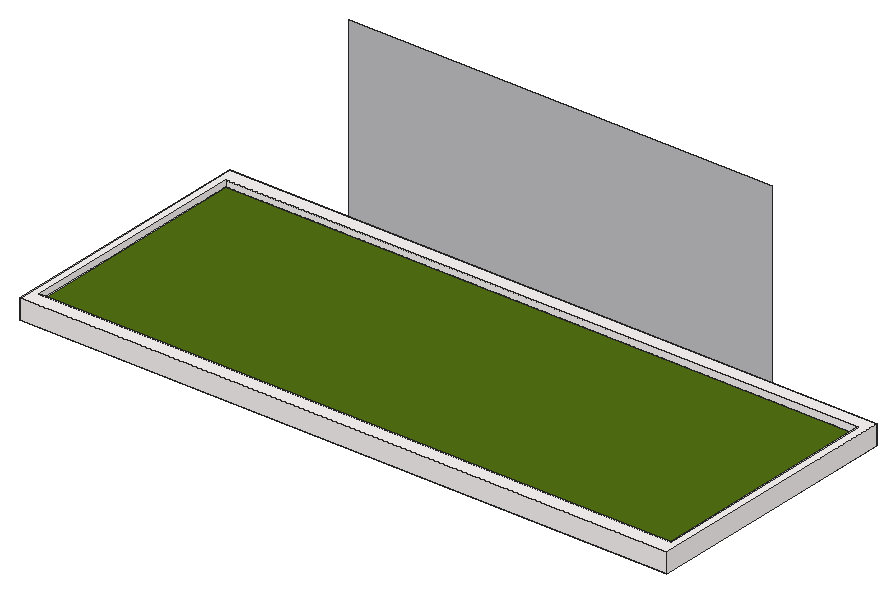
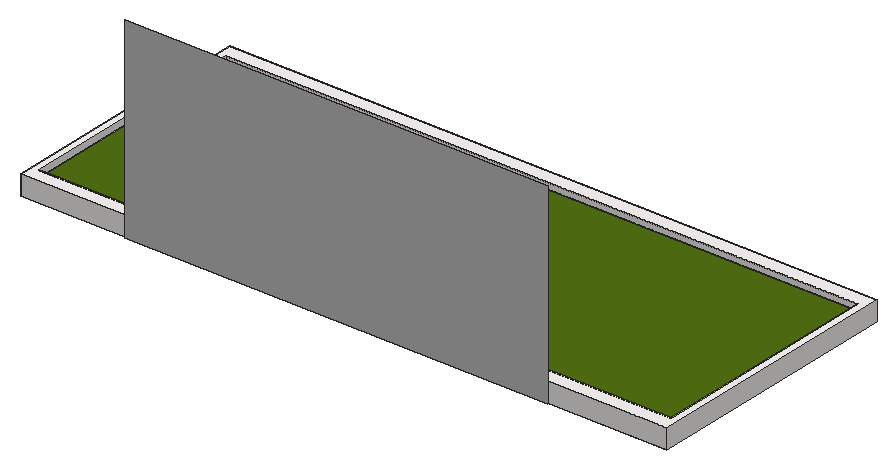
# SketchUp Ruby script. Lengths in inches.
U = 1.inch
M = Sketchup.active_model
def pt(a) = Geom::Point3d.new(a.map { |v| v * U })
def face(e, loops, mat)
  f = e.add_face(loops[0].map { |a| pt(a) })
  loops[1..].each { |l| e.add_face(l.map { |a| pt(a) }).erase! }
  f.material = f.back_material = mat if mat
  f
end
# faces: each face lists its corners as indices into pts; further lists are holes
def faces(e, pts, list, mat = nil) = list.each { |f| face(e, (f[0].is_a?(Array) ? f : [f]).map { |l| l.map { |i| pts[i] } }, mat) }
# xy, xz, yz: faces in a plane at the given z, y or x. An outline is a flat list of corners, or four numbers for a rectangle; further outlines are holes
def ring(l) = l.size == 4 ? [[l[0], l[1]], [l[2], l[1]], [l[2], l[3]], [l[0], l[3]]] : l.each_slice(2).to_a
def flat(e, list, mat, &to3) = list.each { |f| face(e, (f[0].is_a?(Array) ? f : [f]).map { |l| ring(l).map { |u, v| to3.(u, v) } }, mat) }
def xy(e, z, list, mat = nil) = flat(e, list, mat) { |x, y| [x, y, z] }
def xz(e, y, list, mat = nil) = flat(e, list, mat) { |x, z| [x, y, z] }
def yz(e, x, list, mat = nil) = flat(e, list, mat) { |y, z| [x, y, z] }
def lines(e, pts, list) = list.each { |a, b| e.add_line(pt(pts[a]), pt(pts[b])) }
# prism: a flat outline (further loops are holes) pulled along v
def prism(e, loops, v, mat = nil)
  f = face(e, loops, mat); d = Geom::Vector3d.new(v.map { |x| x * U })
  f.pushpull(f.normal.samedirection?(d) ? d.length : -d.length)
end
def box(e, o, s, mat = nil) = prism(e, [[o, [o[0] + s[0], o[1], o[2]], [o[0] + s[0], o[1] + s[1], o[2]], [o[0], o[1] + s[1], o[2]]]], [0, 0, s[2]], mat)
def at(x, y, z, deg = 0) = Geom::Transformation.translation(pt([x, y, z])) * Geom::Transformation.rotation(ORIGIN, Z_AXIS, deg.degrees)
def axes(o, x, y, z) = Geom::Transformation.new([*x, 0, *y, 0, *z, 0, *pt(o).to_a, 1])
def part(name) = M.definitions.add(name)
# library, detail: a bought-in or finely detailed component or shape, given as its bounding box
def library(name, o, s) = part(name).tap { |d| box(d.entities, o, s) }
def detail(e, o, s) = box(e.add_group.entities, o, s)
def put(e, d, t, mat = nil) = e.add_instance(d, t).tap { |i| i.material = mat if mat }
def group(e, t, mat = nil) = e.add_group.tap { |g| g.transformation = t; g.material = mat if mat }.entities
root = M.entities
M.materials.add("[0010_Snow]").color = [255, 250, 250]
M.materials.add("[Polished Concrete New]").color = [200, 200, 203]
M.materials.add("[Vegetation_Blur7]").color = [83, 114, 18]
xy(root,0,[[18.11,15.57,547.58,211.32]])
xy(root,0,[[[11.875,3.95,553.8125,222.94],[18.11,15.57,547.58,211.32]]],"[0010_Snow]")
xy(root,11,[[18.11,15.57,547.58,211.32]],"[Vegetation_Blur7]")
xy(root,16.5,[[[11.875,3.95,553.8125,222.94],[18.11,15.57,547.58,211.32]]],"[0010_Snow]")
xz(root,3.95,[[11.875,0,553.8125,16.5]],"[0010_Snow]")
xz(root,15.57,[[18.11,0,547.58,11],[18.11,11,547.58,16.5]],"[0010_Snow]")
xz(root,211.32,[[18.11,0,547.58,11],[18.11,11,547.58,16.5]],"[0010_Snow]")
xz(root,222.94,[[11.875,0,553.8125,16.5]],"[0010_Snow]")
xz(root,223.5,[[111.625,0,465.4375,163.5625]],"[Polished Concrete New]")
yz(root,11.875,[[3.95,0,222.94,16.5]],"[0010_Snow]")
yz(root,18.11,[[15.57,0,211.32,11],[15.57,11,211.32,16.5]],"[0010_Snow]")
yz(root,547.58,[[15.57,0,211.32,11],[15.57,11,211.32,16.5]],"[0010_Snow]")
yz(root,553.8125,[[3.95,0,222.94,16.5]],"[0010_Snow]")
